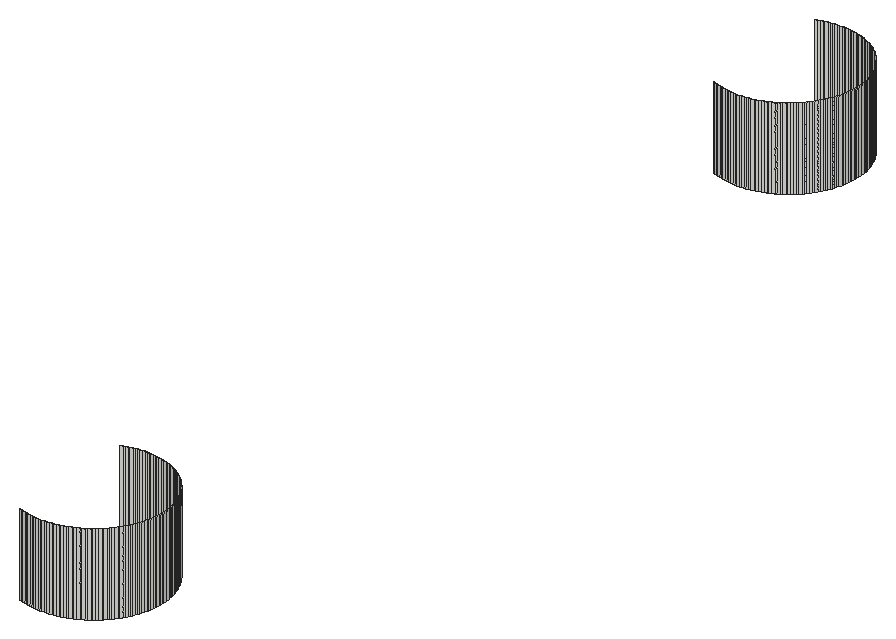
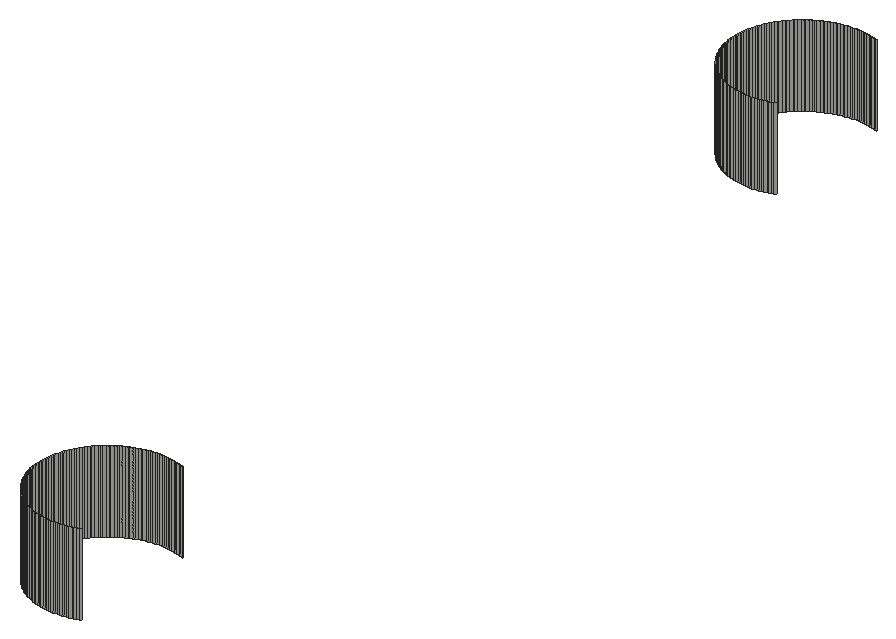
# SketchUp Ruby script. Lengths in inches.
U = 1.inch
M = Sketchup.active_model
def pt(a) = Geom::Point3d.new(a.map { |v| v * U })
def face(e, loops, mat)
  f = e.add_face(loops[0].map { |a| pt(a) })
  loops[1..].each { |l| e.add_face(l.map { |a| pt(a) }).erase! }
  f.material = f.back_material = mat if mat
  f
end
# faces: each face lists its corners as indices into pts; further lists are holes
def faces(e, pts, list, mat = nil) = list.each { |f| face(e, (f[0].is_a?(Array) ? f : [f]).map { |l| l.map { |i| pts[i] } }, mat) }
# xy, xz, yz: faces in a plane at the given z, y or x. An outline is a flat list of corners, or four numbers for a rectangle; further outlines are holes
def ring(l) = l.size == 4 ? [[l[0], l[1]], [l[2], l[1]], [l[2], l[3]], [l[0], l[3]]] : l.each_slice(2).to_a
def flat(e, list, mat, &to3) = list.each { |f| face(e, (f[0].is_a?(Array) ? f : [f]).map { |l| ring(l).map { |u, v| to3.(u, v) } }, mat) }
def xy(e, z, list, mat = nil) = flat(e, list, mat) { |x, y| [x, y, z] }
def xz(e, y, list, mat = nil) = flat(e, list, mat) { |x, z| [x, y, z] }
def yz(e, x, list, mat = nil) = flat(e, list, mat) { |y, z| [x, y, z] }
def lines(e, pts, list) = list.each { |a, b| e.add_line(pt(pts[a]), pt(pts[b])) }
# prism: a flat outline (further loops are holes) pulled along v
def prism(e, loops, v, mat = nil)
  f = face(e, loops, mat); d = Geom::Vector3d.new(v.map { |x| x * U })
  f.pushpull(f.normal.samedirection?(d) ? d.length : -d.length)
end
def box(e, o, s, mat = nil) = prism(e, [[o, [o[0] + s[0], o[1], o[2]], [o[0] + s[0], o[1] + s[1], o[2]], [o[0], o[1] + s[1], o[2]]]], [0, 0, s[2]], mat)
def at(x, y, z, deg = 0) = Geom::Transformation.translation(pt([x, y, z])) * Geom::Transformation.rotation(ORIGIN, Z_AXIS, deg.degrees)
def axes(o, x, y, z) = Geom::Transformation.new([*x, 0, *y, 0, *z, 0, *pt(o).to_a, 1])
def part(name) = M.definitions.add(name)
# library, detail: a bought-in or finely detailed component or shape, given as its bounding box
def library(name, o, s) = part(name).tap { |d| box(d.entities, o, s) }
def detail(e, o, s) = box(e.add_group.entities, o, s)
def put(e, d, t, mat = nil) = e.add_instance(d, t).tap { |i| i.material = mat if mat }
def group(e, t, mat = nil) = e.add_group.tap { |g| g.transformation = t; g.material = mat if mat }.entities
root = M.entities
xz(root,137.5,[[263.84,116,263.92,119],[263.92,116,264,119],[264,116,264.08,119],[264.08,116,264.16,119]])
xz(root,142.5,[[263.84,116,263.92,119],[263.92,116,264,119],[264,116,264.08,119],[264.08,116,264.16,119]])
xz(root,169.5,[[263.84,116,263.92,119],[263.92,116,264,119],[264,116,264.08,119],[264.08,116,264.16,119]])
xz(root,174.5,[[263.84,116,263.92,119],[263.92,116,264,119],[264,116,264.08,119],[264.08,116,264.16,119]])
yz(root,266.49,[[139.76,116,139.84,119],[140.16,116,140.24,119],[171.76,116,171.84,119],[172.16,116,172.24,119]])
yz(root,266.5,[[139.92,116,140,119],[140,116,140.08,119],[171.92,116,172,119],[172,116,172.08,119]])
p = [[263.53,137.54,116],[263.45,137.56,116],[263.45,137.56,119],[263.53,137.54,119],[263.61,137.53,116],[263.61,137.53,119],
  [263.6875,137.52,116],[263.6875,137.52,119],[263.76,137.51,116],[263.76,137.51,119],[263.84,137.5,116],[263.84,137.5,119],
  [264.24,137.51,116],[264.16,137.5,116],[264.16,137.5,119],[264.24,137.51,119],[264.3125,137.52,116],[264.3125,137.52,119],
  [264.39,137.53,116],[264.39,137.53,119],[264.47,137.54,116],[264.47,137.54,119],[264.55,137.56,116],[264.55,137.56,119],
  [263.23,137.62,116],[263.15,137.65,116],[263.15,137.65,119],[263.23,137.62,119],[263.3,137.6,116],[263.3,137.6,119],
  [263.38,137.58,116],[263.38,137.58,119],[264.62,137.58,116],[264.62,137.58,119],[264.7,137.6,116],[264.7,137.6,119],
  [264.77,137.62,116],[264.77,137.62,119],[264.85,137.65,116],[264.85,137.65,119],[264.92,137.68,116],[264.92,137.68,119],
  [264.99,137.71,116],[264.99,137.71,119],[265.0625,137.74,116],[265.0625,137.74,119],[265.13,137.77,116],[265.13,137.77,119],
  [265.2,137.81,116],[265.2,137.81,119],[265.27,137.85,116],[265.27,137.85,119],[265.34,137.89,116],[265.34,137.89,119],
  [265.41,137.93,116],[265.41,137.93,119],[265.47,137.98,116],[265.47,137.98,119],[265.53,138.02,116],[265.53,138.02,119],
  [265.59,138.07,116],[265.59,138.07,119],[265.65,138.125,116],[265.65,138.125,119],[265.71,138.18,116],[265.71,138.18,119],
  [265.77,138.23,116],[265.77,138.23,119],[265.82,138.29,116],[265.82,138.29,119],[265.875,138.35,116],[265.875,138.35,119],
  [265.93,138.41,116],[265.93,138.41,119],[265.98,138.47,116],[265.98,138.47,119],[266.02,138.53,116],[266.02,138.53,119],
  [266.07,138.59,116],[266.07,138.59,119],[266.11,138.66,116],[266.11,138.66,119],[266.15,138.73,116],[266.15,138.73,119],
  [266.19,138.8,116],[266.19,138.8,119],[266.23,138.87,116],[266.23,138.87,119],[266.26,138.9375,116],[266.26,138.9375,119],
  [266.29,139.01,116],[266.29,139.01,119],[266.32,139.08,116],[266.32,139.08,119],[266.35,139.15,116],[266.35,139.15,119],
  [266.38,139.23,116],[266.38,139.23,119],[266.4,139.3,116],[266.4,139.3,119],[266.42,139.38,116],[266.42,139.38,119],
  [266.44,139.45,116],[266.44,139.45,119],[266.46,139.53,116],[266.46,139.53,119],[266.47,139.61,116],[266.47,139.61,119],
  [266.48,139.6875,116],[266.48,139.6875,119],[266.49,139.76,116],[266.49,139.76,119],[266.5,139.92,116],[266.49,139.84,116],
  [266.49,139.84,119],[266.5,139.92,119],[266.49,140.16,116],[266.5,140.08,116],[266.5,140.08,119],[266.49,140.16,119],
  [266.48,140.3125,116],[266.49,140.24,116],[266.49,140.24,119],[266.48,140.3125,119],[266.47,140.39,116],[266.47,140.39,119],
  [266.46,140.47,116],[266.46,140.47,119],[266.42,140.62,116],[266.44,140.55,116],[266.44,140.55,119],[266.42,140.62,119],
  [266.4,140.7,116],[266.4,140.7,119],[266.38,140.77,116],[266.38,140.77,119],[266.32,140.92,116],[266.35,140.85,116],
  [266.35,140.85,119],[266.32,140.92,119],[266.29,140.99,116],[266.29,140.99,119],[266.26,141.0625,116],[266.26,141.0625,119],
  [266.19,141.2,116],[266.23,141.13,116],[266.23,141.13,119],[266.19,141.2,119],[266.15,141.27,116],[266.15,141.27,119],
  [266.07,141.41,116],[266.11,141.34,116],[266.11,141.34,119],[266.07,141.41,119],[266.02,141.47,116],[266.02,141.47,119],
  [265.93,141.59,116],[265.98,141.53,116],[265.98,141.53,119],[265.93,141.59,119],[265.875,141.65,116],[265.875,141.65,119],
  [265.77,141.77,116],[265.82,141.71,116],[265.82,141.71,119],[265.77,141.77,119],[265.65,141.875,116],[265.71,141.82,116],
  [265.71,141.82,119],[265.65,141.875,119],[265.53,141.98,116],[265.59,141.93,116],[265.59,141.93,119],[265.53,141.98,119],
  [265.41,142.07,116],[265.47,142.02,116],[265.47,142.02,119],[265.41,142.07,119],[265.27,142.15,116],[265.34,142.11,116],
  [265.34,142.11,119],[265.27,142.15,119],[265.0625,142.26,116],[265.13,142.23,116],[265.13,142.23,119],[265.0625,142.26,119],
  [265.2,142.19,116],[265.2,142.19,119],[263.08,142.32,116],[263.15,142.35,116],[263.15,142.35,119],[263.08,142.32,119],
  [264.85,142.35,116],[264.92,142.32,116],[264.92,142.32,119],[264.85,142.35,119],[264.99,142.29,116],[264.99,142.29,119],
  [263.23,142.38,116],[263.23,142.38,119],[263.3,142.4,116],[263.3,142.4,119],[263.38,142.42,116],[263.38,142.42,119],
  [263.45,142.44,116],[263.45,142.44,119],[263.53,142.46,116],[263.53,142.46,119],[264.47,142.46,116],[264.55,142.44,116],
  [264.55,142.44,119],[264.47,142.46,119],[264.62,142.42,116],[264.62,142.42,119],[264.7,142.4,116],[264.7,142.4,119],
  [264.77,142.38,116],[264.77,142.38,119],[263.61,142.47,116],[263.61,142.47,119],[263.6875,142.48,116],[263.6875,142.48,119],
  [263.76,142.49,116],[263.76,142.49,119],[263.84,142.5,116],[263.84,142.5,119],[264.16,142.5,116],[264.24,142.49,116],
  [264.24,142.49,119],[264.16,142.5,119],[264.3125,142.48,116],[264.3125,142.48,119],[264.39,142.47,116],[264.39,142.47,119],
  [263.53,169.54,116],[263.45,169.56,116],[263.45,169.56,119],[263.53,169.54,119],[263.61,169.53,116],[263.61,169.53,119],
  [263.6875,169.52,116],[263.6875,169.52,119],[263.76,169.51,116],[263.76,169.51,119],[263.84,169.5,116],[263.84,169.5,119],
  [264.24,169.51,116],[264.16,169.5,116],[264.16,169.5,119],[264.24,169.51,119],[264.3125,169.52,116],[264.3125,169.52,119],
  [264.39,169.53,116],[264.39,169.53,119],[264.47,169.54,116],[264.47,169.54,119],[264.55,169.56,116],[264.55,169.56,119],
  [263.15,169.65,116],[263.08,169.68,116],[263.08,169.68,119],[263.15,169.65,119],[263.23,169.62,116],[263.23,169.62,119],
  [263.3,169.6,116],[263.3,169.6,119],[263.38,169.58,116],[263.38,169.58,119],[264.62,169.58,116],[264.62,169.58,119],
  [264.7,169.6,116],[264.7,169.6,119],[264.77,169.62,116],[264.77,169.62,119],[264.85,169.65,116],[264.85,169.65,119],
  [264.92,169.68,116],[264.92,169.68,119],[264.99,169.71,116],[264.99,169.71,119],[265.0625,169.74,116],[265.0625,169.74,119],
  [265.13,169.77,116],[265.13,169.77,119],[265.2,169.81,116],[265.2,169.81,119],[265.27,169.85,116],[265.27,169.85,119],
  [265.34,169.89,116],[265.34,169.89,119],[265.41,169.93,116],[265.41,169.93,119],[265.47,169.98,116],[265.47,169.98,119],
  [265.53,170.02,116],[265.53,170.02,119],[265.59,170.07,116],[265.59,170.07,119],[265.65,170.125,116],[265.65,170.125,119],
  [265.71,170.18,116],[265.71,170.18,119],[265.77,170.23,116],[265.77,170.23,119],[265.82,170.29,116],[265.82,170.29,119],
  [265.875,170.35,116],[265.875,170.35,119],[265.93,170.41,116],[265.93,170.41,119],[265.98,170.47,116],[265.98,170.47,119],
  [266.02,170.53,116],[266.02,170.53,119],[266.07,170.59,116],[266.07,170.59,119],[266.11,170.66,116],[266.11,170.66,119],
  [266.15,170.73,116],[266.15,170.73,119],[266.19,170.8,116],[266.19,170.8,119],[266.23,170.87,116],[266.23,170.87,119],
  [266.26,170.9375,116],[266.26,170.9375,119],[266.29,171.01,116],[266.29,171.01,119],[266.32,171.08,116],[266.32,171.08,119],
  [266.35,171.15,116],[266.35,171.15,119],[266.38,171.23,116],[266.38,171.23,119],[266.4,171.3,116],[266.4,171.3,119],
  [266.42,171.38,116],[266.42,171.38,119],[266.44,171.45,116],[266.44,171.45,119],[266.46,171.53,116],[266.46,171.53,119],
  [266.47,171.61,116],[266.47,171.61,119],[266.48,171.6875,116],[266.48,171.6875,119],[266.49,171.76,116],[266.49,171.76,119],
  [266.5,171.92,116],[266.49,171.84,116],[266.49,171.84,119],[266.5,171.92,119],[266.49,172.16,116],[266.5,172.08,116],
  [266.5,172.08,119],[266.49,172.16,119],[266.48,172.3125,116],[266.49,172.24,116],[266.49,172.24,119],[266.48,172.3125,119],
  [266.47,172.39,116],[266.47,172.39,119],[266.46,172.47,116],[266.46,172.47,119],[266.42,172.62,116],[266.44,172.55,116],
  [266.44,172.55,119],[266.42,172.62,119],[266.4,172.7,116],[266.4,172.7,119],[266.38,172.77,116],[266.38,172.77,119],
  [266.32,172.92,116],[266.35,172.85,116],[266.35,172.85,119],[266.32,172.92,119],[266.29,172.99,116],[266.29,172.99,119],
  [266.26,173.0625,116],[266.26,173.0625,119],[266.19,173.2,116],[266.23,173.13,116],[266.23,173.13,119],[266.19,173.2,119],
  [266.15,173.27,116],[266.15,173.27,119],[266.07,173.41,116],[266.11,173.34,116],[266.11,173.34,119],[266.07,173.41,119],
  [266.02,173.47,116],[266.02,173.47,119],[265.93,173.59,116],[265.98,173.53,116],[265.98,173.53,119],[265.93,173.59,119],
  [265.875,173.65,116],[265.875,173.65,119],[265.77,173.77,116],[265.82,173.71,116],[265.82,173.71,119],[265.77,173.77,119],
  [265.65,173.875,116],[265.71,173.82,116],[265.71,173.82,119],[265.65,173.875,119],[265.53,173.98,116],[265.59,173.93,116],
  [265.59,173.93,119],[265.53,173.98,119],[265.41,174.07,116],[265.47,174.02,116],[265.47,174.02,119],[265.41,174.07,119],
  [265.27,174.15,116],[265.34,174.11,116],[265.34,174.11,119],[265.27,174.15,119],[265.0625,174.26,116],[265.13,174.23,116],
  [265.13,174.23,119],[265.0625,174.26,119],[265.2,174.19,116],[265.2,174.19,119],[263.08,174.32,116],[263.15,174.35,116],
  [263.15,174.35,119],[263.08,174.32,119],[264.85,174.35,116],[264.92,174.32,116],[264.92,174.32,119],[264.85,174.35,119],
  [264.99,174.29,116],[264.99,174.29,119],[263.23,174.38,116],[263.23,174.38,119],[263.3,174.4,116],[263.3,174.4,119],
  [263.38,174.42,116],[263.38,174.42,119],[263.45,174.44,116],[263.45,174.44,119],[263.53,174.46,116],[263.53,174.46,119],
  [264.47,174.46,116],[264.55,174.44,116],[264.55,174.44,119],[264.47,174.46,119],[264.62,174.42,116],[264.62,174.42,119],
  [264.7,174.4,116],[264.7,174.4,119],[264.77,174.38,116],[264.77,174.38,119],[263.61,174.47,116],[263.61,174.47,119],
  [263.6875,174.48,116],[263.6875,174.48,119],[263.76,174.49,116],[263.76,174.49,119],[263.84,174.5,116],[263.84,174.5,119],
  [264.16,174.5,116],[264.24,174.49,116],[264.24,174.49,119],[264.16,174.5,119],[264.3125,174.48,116],[264.3125,174.48,119],
  [264.39,174.47,116],[264.39,174.47,119]]
faces(root,p,[[0,1,2,3],[4,0,3,5],[6,4,5,7],[8,6,7,9],[10,8,9,11],[12,13,14,15],[16,12,15,17],[18,16,17,19],
  [20,18,19,21],[22,20,21,23],[24,25,26,27],[28,24,27,29],[30,28,29,31],[1,30,31,2],[32,22,23,33],[34,32,33,35],
  [36,34,35,37],[38,36,37,39],[40,38,39,41],[42,40,41,43],[44,42,43,45],[46,44,45,47],[48,46,47,49],[50,48,49,51],
  [52,50,51,53],[54,52,53,55],[56,54,55,57],[58,56,57,59],[60,58,59,61],[62,60,61,63],[64,62,63,65],[66,64,65,67],
  [68,66,67,69],[70,68,69,71],[72,70,71,73],[74,72,73,75],[76,74,75,77],[78,76,77,79],[80,78,79,81],[82,80,81,83],
  [84,82,83,85],[86,84,85,87],[88,86,87,89],[90,88,89,91],[92,90,91,93],[94,92,93,95],[96,94,95,97],[98,96,97,99],
  [100,98,99,101],[102,100,101,103],[104,102,103,105],[106,104,105,107],[108,106,107,109],[110,108,109,111],[112,113,114,115],[116,117,118,119],
  [120,121,122,123],[124,120,123,125],[126,124,125,127],[128,129,130,131],[129,126,127,130],[132,128,131,133],[134,132,133,135],[136,137,138,139],
  [137,134,135,138],[140,136,139,141],[142,140,141,143],[144,145,146,147],[145,142,143,146],[148,144,147,149],[150,151,152,153],[151,148,149,152],
  [154,150,153,155],[156,157,158,159],[157,154,155,158],[160,156,159,161],[162,163,164,165],[163,160,161,164],[166,167,168,169],[167,162,165,168],
  [170,171,172,173],[171,166,169,172],[174,175,176,177],[175,170,173,176],[178,179,180,181],[179,174,177,180],[182,183,184,185],[183,186,187,184],
  [186,178,181,187],[188,189,190,191],[192,193,194,195],[193,196,197,194],[196,182,185,197],[189,198,199,190],[198,200,201,199],[200,202,203,201],
  [202,204,205,203],[204,206,207,205],[208,209,210,211],[209,212,213,210],[212,214,215,213],[214,216,217,215],[216,192,195,217],[206,218,219,207],
  [218,220,221,219],[220,222,223,221],[222,224,225,223],[226,227,228,229],[227,230,231,228],[230,232,233,231],[232,208,211,233],[234,235,236,237],
  [238,234,237,239],[240,238,239,241],[242,240,241,243],[244,242,243,245],[246,247,248,249],[250,246,249,251],[252,250,251,253],[254,252,253,255],
  [256,254,255,257],[258,259,260,261],[262,258,261,263],[264,262,263,265],[266,264,265,267],[235,266,267,236],[268,256,257,269],[270,268,269,271],
  [272,270,271,273],[274,272,273,275],[276,274,275,277],[278,276,277,279],[280,278,279,281],[282,280,281,283],[284,282,283,285],[286,284,285,287],
  [288,286,287,289],[290,288,289,291],[292,290,291,293],[294,292,293,295],[296,294,295,297],[298,296,297,299],[300,298,299,301],[302,300,301,303],
  [304,302,303,305],[306,304,305,307],[308,306,307,309],[310,308,309,311],[312,310,311,313],[314,312,313,315],[316,314,315,317],[318,316,317,319],
  [320,318,319,321],[322,320,321,323],[324,322,323,325],[326,324,325,327],[328,326,327,329],[330,328,329,331],[332,330,331,333],[334,332,333,335],
  [336,334,335,337],[338,336,337,339],[340,338,339,341],[342,340,341,343],[344,342,343,345],[346,344,345,347],[348,349,350,351],[352,353,354,355],
  [356,357,358,359],[360,356,359,361],[362,360,361,363],[364,365,366,367],[365,362,363,366],[368,364,367,369],[370,368,369,371],[372,373,374,375],
  [373,370,371,374],[376,372,375,377],[378,376,377,379],[380,381,382,383],[381,378,379,382],[384,380,383,385],[386,387,388,389],[387,384,385,388],
  [390,386,389,391],[392,393,394,395],[393,390,391,394],[396,392,395,397],[398,399,400,401],[399,396,397,400],[402,403,404,405],[403,398,401,404],
  [406,407,408,409],[407,402,405,408],[410,411,412,413],[411,406,409,412],[414,415,416,417],[415,410,413,416],[418,419,420,421],[419,422,423,420],
  [422,414,417,423],[424,425,426,427],[428,429,430,431],[429,432,433,430],[432,418,421,433],[425,434,435,426],[434,436,437,435],[436,438,439,437],
  [438,440,441,439],[440,442,443,441],[444,445,446,447],[445,448,449,446],[448,450,451,449],[450,452,453,451],[452,428,431,453],[442,454,455,443],
  [454,456,457,455],[456,458,459,457],[458,460,461,459],[462,463,464,465],[463,466,467,464],[466,468,469,467],[468,444,447,469]])
